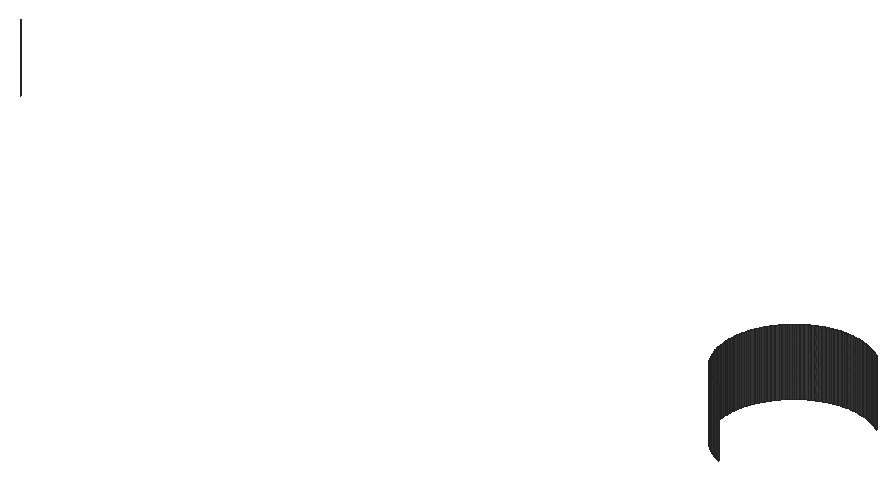
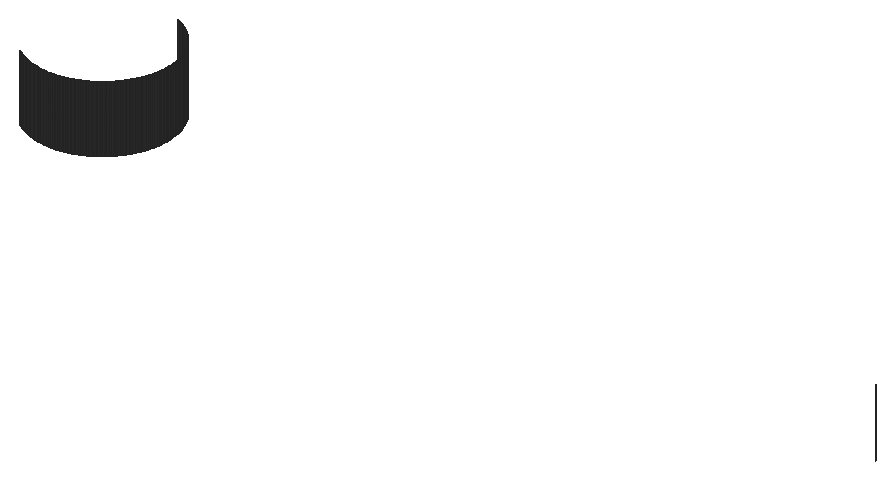
# SketchUp Ruby script. Lengths in inches.
U = 1.inch
M = Sketchup.active_model
def pt(a) = Geom::Point3d.new(a.map { |v| v * U })
def face(e, loops, mat)
  f = e.add_face(loops[0].map { |a| pt(a) })
  loops[1..].each { |l| e.add_face(l.map { |a| pt(a) }).erase! }
  f.material = f.back_material = mat if mat
  f
end
# faces: each face lists its corners as indices into pts; further lists are holes
def faces(e, pts, list, mat = nil) = list.each { |f| face(e, (f[0].is_a?(Array) ? f : [f]).map { |l| l.map { |i| pts[i] } }, mat) }
# xy, xz, yz: faces in a plane at the given z, y or x. An outline is a flat list of corners, or four numbers for a rectangle; further outlines are holes
def ring(l) = l.size == 4 ? [[l[0], l[1]], [l[2], l[1]], [l[2], l[3]], [l[0], l[3]]] : l.each_slice(2).to_a
def flat(e, list, mat, &to3) = list.each { |f| face(e, (f[0].is_a?(Array) ? f : [f]).map { |l| ring(l).map { |u, v| to3.(u, v) } }, mat) }
def xy(e, z, list, mat = nil) = flat(e, list, mat) { |x, y| [x, y, z] }
def xz(e, y, list, mat = nil) = flat(e, list, mat) { |x, z| [x, y, z] }
def yz(e, x, list, mat = nil) = flat(e, list, mat) { |y, z| [x, y, z] }
def lines(e, pts, list) = list.each { |a, b| e.add_line(pt(pts[a]), pt(pts[b])) }
# prism: a flat outline (further loops are holes) pulled along v
def prism(e, loops, v, mat = nil)
  f = face(e, loops, mat); d = Geom::Vector3d.new(v.map { |x| x * U })
  f.pushpull(f.normal.samedirection?(d) ? d.length : -d.length)
end
def box(e, o, s, mat = nil) = prism(e, [[o, [o[0] + s[0], o[1], o[2]], [o[0] + s[0], o[1] + s[1], o[2]], [o[0], o[1] + s[1], o[2]]]], [0, 0, s[2]], mat)
def at(x, y, z, deg = 0) = Geom::Transformation.translation(pt([x, y, z])) * Geom::Transformation.rotation(ORIGIN, Z_AXIS, deg.degrees)
def axes(o, x, y, z) = Geom::Transformation.new([*x, 0, *y, 0, *z, 0, *pt(o).to_a, 1])
def part(name) = M.definitions.add(name)
# library, detail: a bought-in or finely detailed component or shape, given as its bounding box
def library(name, o, s) = part(name).tap { |d| box(d.entities, o, s) }
def detail(e, o, s) = box(e.add_group.entities, o, s)
def put(e, d, t, mat = nil) = e.add_instance(d, t).tap { |i| i.material = mat if mat }
def group(e, t, mat = nil) = e.add_group.tap { |g| g.transformation = t; g.material = mat if mat }.entities
root = M.entities
M.materials.add("1448 AP 8253 RAVEN SONG").color = [64, 64, 63]
xz(root,209.99,[[77.68,120,77.76,123],[78.15,120,78.23,123]],"1448 AP 8253 RAVEN SONG")
xz(root,210,[[77.83,120,77.91,123],[77.91,120,77.99,123],[77.99,120,78.07,123]],"1448 AP 8253 RAVEN SONG")
yz(root,74.97,[[206.86,120,206.94,123],[206.94,120,207.02,123],[207.02,120,207.1,123]],"1448 AP 8253 RAVEN SONG")
yz(root,74.98,[[206.71,120,206.79,123],[207.18,120,207.26,123]],"1448 AP 8253 RAVEN SONG")
p = [[76.8,204.24,120],[76.73,204.27,120],[76.73,204.27,123],[76.8,204.24,123],[76.59,204.34,120],[76.52,204.375,120],
  [76.52,204.375,123],[76.59,204.34,123],[76.66,204.3,120],[76.66,204.3,123],[76.45,204.41,120],[76.39,204.45,120],
  [76.39,204.45,123],[76.45,204.41,123],[76.25,204.54,120],[76.19,204.59,120],[76.19,204.59,123],[76.25,204.54,123],
  [76.32,204.5,120],[76.32,204.5,123],[76.13,204.63,120],[76.13,204.63,123],[76.07,204.68,120],[76.07,204.68,123],
  [76.01,204.73,120],[75.95,204.78,120],[75.95,204.78,123],[76.01,204.73,123],[75.89,204.84,120],[75.83,204.89,120],
  [75.83,204.89,123],[75.89,204.84,123],[75.78,204.95,120],[75.73,205.01,120],[75.73,205.01,123],[75.78,204.95,123],
  [75.68,205.07,120],[75.68,205.07,123],[75.625,205.13,120],[75.625,205.13,123],[75.58,205.19,120],[75.58,205.19,123],
  [75.53,205.25,120],[75.53,205.25,123],[75.49,205.32,120],[75.44,205.38,120],[75.44,205.38,123],[75.49,205.32,123],
  [75.4,205.45,120],[75.4,205.45,123],[75.36,205.52,120],[75.32,205.59,120],[75.32,205.59,123],[75.36,205.52,123],
  [75.29,205.66,120],[75.29,205.66,123],[75.25,205.73,120],[75.22,205.8,120],[75.22,205.8,123],[75.25,205.73,123],
  [75.19,205.87,120],[75.19,205.87,123],[75.16,205.94,120],[75.14,206.02,120],[75.14,206.02,123],[75.16,205.94,123],
  [75.11,206.09,120],[75.11,206.09,123],[75.09,206.17,120],[75.09,206.17,123],[75.07,206.24,120],[75.05,206.32,120],
  [75.05,206.32,123],[75.07,206.24,123],[75.03,206.4,120],[75.03,206.4,123],[75.02,206.47,120],[75.02,206.47,123],
  [75,206.55,120],[75,206.55,123],[74.99,206.63,120],[74.99,206.63,123],[74.98,206.71,120],[74.98,206.71,123],
  [74.98,206.79,120],[74.97,206.86,120],[74.97,206.86,123],[74.98,206.79,123],[74.97,207.1,120],[74.98,207.18,120],
  [74.98,207.18,123],[74.97,207.1,123],[74.98,207.26,120],[74.99,207.33,120],[74.99,207.33,123],[74.98,207.26,123],
  [75,207.41,120],[75,207.41,123],[75.01,207.49,120],[75.01,207.49,123],[75.02,207.57,120],[75.02,207.57,123],
  [75.04,207.64,120],[75.04,207.64,123],[75.06,207.72,120],[75.06,207.72,123],[75.08,207.8,120],[75.08,207.8,123],
  [75.1,207.87,120],[75.1,207.87,123],[75.125,207.95,120],[75.125,207.95,123],[75.15,208.02,120],[75.15,208.02,123],
  [75.18,208.09,120],[75.18,208.09,123],[75.21,208.17,120],[75.21,208.17,123],[75.24,208.24,120],[75.24,208.24,123],
  [75.27,208.31,120],[75.27,208.31,123],[75.31,208.38,120],[75.31,208.38,123],[75.34,208.45,120],[75.34,208.45,123],
  [75.38,208.52,120],[75.38,208.52,123],[75.42,208.58,120],[75.42,208.58,123],[75.47,208.65,120],[75.47,208.65,123],
  [75.51,208.72,120],[75.51,208.72,123],[75.56,208.78,120],[75.56,208.78,123],[75.6,208.84,120],[75.6,208.84,123],
  [75.65,208.9,120],[75.65,208.9,123],[75.7,208.96,120],[75.7,208.96,123],[75.75,209.02,120],[75.75,209.02,123],
  [75.81,209.08,120],[75.81,209.08,123],[75.86,209.14,120],[75.86,209.14,123],[75.92,209.19,120],[75.92,209.19,123],
  [75.98,209.24,120],[75.98,209.24,123],[76.04,209.29,120],[76.04,209.29,123],[76.1,209.34,120],[76.1,209.34,123],
  [76.16,209.39,120],[76.16,209.39,123],[41.23,209.41,120],[41.29,209.37,120],[41.29,209.37,123],[41.23,209.41,123],
  [76.22,209.4375,120],[76.22,209.4375,123],[76.29,209.48,120],[76.29,209.48,123],[79.6875,209.46,120],[79.75,209.41,120],
  [79.75,209.41,123],[79.6875,209.46,123],[76.35,209.53,120],[76.35,209.53,123],[76.42,209.57,120],[76.42,209.57,123],
  [79.49,209.59,120],[79.55,209.55,120],[79.55,209.55,123],[79.49,209.59,123],[79.62,209.5,120],[79.62,209.5,123],
  [76.49,209.61,120],[76.49,209.61,123],[76.56,209.65,120],[76.56,209.65,123],[76.625,209.68,120],[76.625,209.68,123],
  [79.35,209.66,120],[79.42,209.625,120],[79.42,209.625,123],[79.35,209.66,123],[76.7,209.72,120],[76.7,209.72,123],
  [76.77,209.75,120],[76.77,209.75,123],[76.84,209.78,120],[76.84,209.78,123],[79.14,209.76,120],[79.21,209.73,120],
  [79.21,209.73,123],[79.14,209.76,123],[79.28,209.7,120],[79.28,209.7,123],[76.91,209.81,120],[76.91,209.81,123],
  [76.99,209.83,120],[76.99,209.83,123],[77.0625,209.86,120],[77.0625,209.86,123],[78.84,209.87,120],[78.92,209.85,120],
  [78.92,209.85,123],[78.84,209.87,123],[78.99,209.82,120],[78.99,209.82,123],[79.0625,209.79,120],[79.0625,209.79,123],
  [77.14,209.88,120],[77.14,209.88,123],[77.21,209.9,120],[77.21,209.9,123],[77.29,209.92,120],[77.29,209.92,123],
  [77.37,209.9375,120],[77.37,209.9375,123],[77.44,209.95,120],[77.44,209.95,123],[78.46,209.96,120],[78.54,209.95,120],
  [78.54,209.95,123],[78.46,209.96,123],[78.61,209.93,120],[78.61,209.93,123],[78.69,209.91,120],[78.69,209.91,123],
  [78.77,209.89,120],[78.77,209.89,123],[77.52,209.97,120],[77.52,209.97,123],[77.6,209.98,120],[77.6,209.98,123],
  [77.68,209.99,120],[77.68,209.99,123],[77.76,209.99,120],[77.83,210,120],[77.83,210,123],[77.76,209.99,123],
  [78.07,210,120],[78.15,209.99,120],[78.15,209.99,123],[78.07,210,123],[78.23,209.99,120],[78.3,209.98,120],
  [78.3,209.98,123],[78.23,209.99,123],[78.38,209.97,120],[78.38,209.97,123]]
faces(root,p,[[0,1,2,3],[4,5,6,7],[8,4,7,9],[1,8,9,2],[10,11,12,13],[5,10,13,6],[14,15,16,17],[11,18,19,12],
  [18,14,17,19],[15,20,21,16],[20,22,23,21],[24,25,26,27],[22,24,27,23],[28,29,30,31],[25,28,31,26],[32,33,34,35],
  [29,32,35,30],[33,36,37,34],[36,38,39,37],[38,40,41,39],[40,42,43,41],[44,45,46,47],[42,44,47,43],[45,48,49,46],
  [50,51,52,53],[48,50,53,49],[51,54,55,52],[56,57,58,59],[54,56,59,55],[57,60,61,58],[62,63,64,65],[60,62,65,61],
  [63,66,67,64],[66,68,69,67],[70,71,72,73],[68,70,73,69],[71,74,75,72],[74,76,77,75],[76,78,79,77],[78,80,81,79],
  [80,82,83,81],[84,85,86,87],[88,89,90,91],[92,93,94,95],[93,96,97,94],[96,98,99,97],[98,100,101,99],[100,102,103,101],
  [102,104,105,103],[104,106,107,105],[106,108,109,107],[108,110,111,109],[110,112,113,111],[112,114,115,113],[114,116,117,115],[116,118,119,117],
  [118,120,121,119],[120,122,123,121],[122,124,125,123],[124,126,127,125],[126,128,129,127],[128,130,131,129],[130,132,133,131],[132,134,135,133],
  [134,136,137,135],[136,138,139,137],[138,140,141,139],[140,142,143,141],[142,144,145,143],[144,146,147,145],[146,148,149,147],[148,150,151,149],
  [150,152,153,151],[152,154,155,153],[154,156,157,155],[158,159,160,161],[156,162,163,157],[162,164,165,163],[166,167,168,169],[164,170,171,165],
  [170,172,173,171],[174,175,176,177],[175,178,179,176],[178,166,169,179],[172,180,181,173],[180,182,183,181],[182,184,185,183],[186,187,188,189],
  [187,174,177,188],[184,190,191,185],[190,192,193,191],[192,194,195,193],[196,197,198,199],[197,200,201,198],[200,186,189,201],[194,202,203,195],
  [202,204,205,203],[204,206,207,205],[208,209,210,211],[209,212,213,210],[212,214,215,213],[214,196,199,215],[206,216,217,207],[216,218,219,217],
  [218,220,221,219],[220,222,223,221],[222,224,225,223],[226,227,228,229],[227,230,231,228],[230,232,233,231],[232,234,235,233],[234,208,211,235],
  [224,236,237,225],[236,238,239,237],[238,240,241,239],[242,243,244,245],[246,247,248,249],[250,251,252,253],[251,254,255,252],[254,226,229,255]],"1448 AP 8253 RAVEN SONG")
